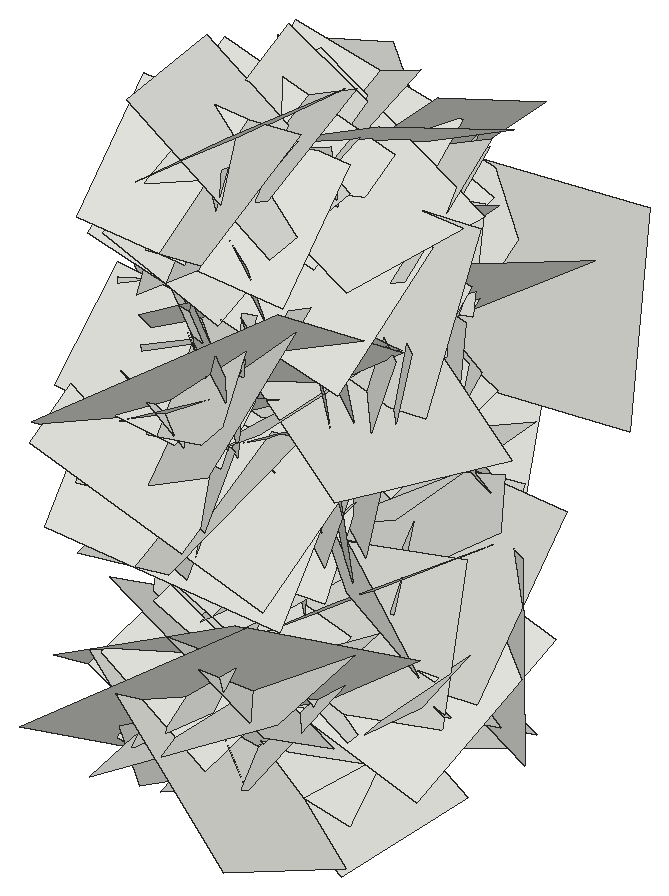
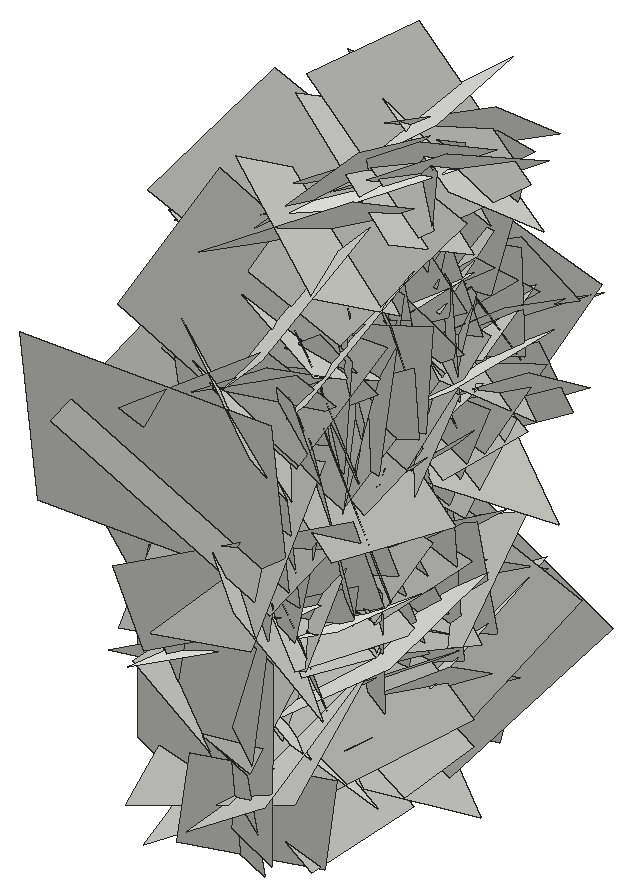
# SketchUp Ruby script. Lengths in inches.
U = 1.inch
M = Sketchup.active_model
def pt(a) = Geom::Point3d.new(a.map { |v| v * U })
def face(e, loops, mat)
  f = e.add_face(loops[0].map { |a| pt(a) })
  loops[1..].each { |l| e.add_face(l.map { |a| pt(a) }).erase! }
  f.material = f.back_material = mat if mat
  f
end
# faces: each face lists its corners as indices into pts; further lists are holes
def faces(e, pts, list, mat = nil) = list.each { |f| face(e, (f[0].is_a?(Array) ? f : [f]).map { |l| l.map { |i| pts[i] } }, mat) }
# xy, xz, yz: faces in a plane at the given z, y or x. An outline is a flat list of corners, or four numbers for a rectangle; further outlines are holes
def ring(l) = l.size == 4 ? [[l[0], l[1]], [l[2], l[1]], [l[2], l[3]], [l[0], l[3]]] : l.each_slice(2).to_a
def flat(e, list, mat, &to3) = list.each { |f| face(e, (f[0].is_a?(Array) ? f : [f]).map { |l| ring(l).map { |u, v| to3.(u, v) } }, mat) }
def xy(e, z, list, mat = nil) = flat(e, list, mat) { |x, y| [x, y, z] }
def xz(e, y, list, mat = nil) = flat(e, list, mat) { |x, z| [x, y, z] }
def yz(e, x, list, mat = nil) = flat(e, list, mat) { |y, z| [x, y, z] }
def lines(e, pts, list) = list.each { |a, b| e.add_line(pt(pts[a]), pt(pts[b])) }
# prism: a flat outline (further loops are holes) pulled along v
def prism(e, loops, v, mat = nil)
  f = face(e, loops, mat); d = Geom::Vector3d.new(v.map { |x| x * U })
  f.pushpull(f.normal.samedirection?(d) ? d.length : -d.length)
end
def box(e, o, s, mat = nil) = prism(e, [[o, [o[0] + s[0], o[1], o[2]], [o[0] + s[0], o[1] + s[1], o[2]], [o[0], o[1] + s[1], o[2]]]], [0, 0, s[2]], mat)
def at(x, y, z, deg = 0) = Geom::Transformation.translation(pt([x, y, z])) * Geom::Transformation.rotation(ORIGIN, Z_AXIS, deg.degrees)
def axes(o, x, y, z) = Geom::Transformation.new([*x, 0, *y, 0, *z, 0, *pt(o).to_a, 1])
def part(name) = M.definitions.add(name)
# library, detail: a bought-in or finely detailed component or shape, given as its bounding box
def library(name, o, s) = part(name).tap { |d| box(d.entities, o, s) }
def detail(e, o, s) = box(e.add_group.entities, o, s)
def put(e, d, t, mat = nil) = e.add_instance(d, t).tap { |i| i.material = mat if mat }
def group(e, t, mat = nil) = e.add_group.tap { |g| g.transformation = t; g.material = mat if mat }.entities
root = M.entities
c1 = part("Component\#6")
p = [[0.01,0,0],[0,3.24,4.54],[4.32,3.24,4.54],[4.33,0,0]]
faces(c1.entities,p,[[0,1,2,3]])
put(root,c1,axes([420.52,211.4,20.36],[-0.11841,0.02386,0.67628],[0.07272,0.6823,-0.01274],[0.7136,-0.06557,0.11352]))
put(root,c1,axes([420.52,208.95,27.68],[-0.1117,0.11156,-0.75397],[-0.06454,-0.75994,-0.10393],[0.80532,-0.04543,-0.11291]))
put(root,c1,axes([420.52,203.96,20.97],[0.02025,-0.24988,0.58047],[-0.03388,0.57961,0.25056],[0.66903,0.03691,-0.00488]))
put(root,c1,axes([420.52,202.42,34.22],[-0.03507,0.56649,-0.26791],[0.06705,-0.26389,-0.56581],[0.66085,0.05684,0.04319]))
put(root,c1,axes([424.49,211.47,22.62],[0.20513,-1.22241,0.07319],[0.04122,0.08019,1.23659],[-1.29742,-0.19072,0.05085]))
put(root,c1,axes([424.49,206.36,33.23],[0.09168,1.1059,0.20164],[0.04784,0.19866,-1.1089],[-1.19063,0.09314,-0.02903]))
put(root,c1,axes([424.49,205.67,24.52],[-0.15369,0.87531,0.08009],[0.01982,0.08422,-0.88666],[-0.9315,-0.14262,-0.03208]))
put(root,c1,axes([424.49,207.21,30.03],[0.00943,-1.01637,-0.0193],[0.00822,-0.01923,1.01638],[-1.07752,-0.00904,0.00758]))
put(root,c1,axes([420.52,204.95,35.05],[0.03568,0.1968,-0.61743],[-0.04358,-0.61637,-0.1987],[0.68554,-0.04943,0.01951]))
put(root,c1,axes([420.52,212.36,26.625],[-0.06935,-0.64087,-0.11796],[0.11905,-0.12787,0.63241],[0.68039,-0.04294,-0.12268]))
put(root,c1,axes([420.52,206.625,39.5],[-0.00312,0.09172,-0.66161],[0.00201,-0.66161,-0.09173],[0.70801,0.00228,-0.00265]))
put(root,c1,axes([420.52,204.22,36.67],[0.08595,0.41822,-0.43473],[-0.01861,-0.43682,-0.42351],[0.63917,-0.06896,0.04613]))
put(root,c1,axes([420.52,202.23,33.91],[0.02493,0.60398,0.49928],[-0.17768,0.49182,-0.58706],[0.81142,0.08914,-0.14389]))
put(root,c1,axes([420.52,200.85,29.625],[-0.04324,0.39016,0.69087],[-0.10275,0.68414,-0.39209],[0.83473,0.10443,-0.01247]))
put(root,c1,axes([420.52,212.78,35.18],[-0.06835,-0.19577,-0.64021],[0.13077,-0.63563,0.18195],[0.69749,0.09999,-0.09685]))
put(root,c1,axes([420.52,211.1,35.2],[0.07899,0.5337,0.27791],[0.02897,0.27674,-0.53878],[0.63716,-0.07875,-0.00996]))
put(root,c1,axes([424.49,202.75,27.49],[0.17368,0.85862,-0.51485],[-0.1903,-0.48804,-0.87105],[-1.04401,0.2318,0.07312]))
put(root,c1,axes([420.52,206.77,29.69],[0.13468,0.0618,0.68245],[-0.14259,0.68282,-0.03679],[0.71222,0.12502,-0.13642]))
put(root,c1,axes([424.49,204.74,34.65],[-0.08046,-0.48471,-0.63269],[-0.12911,-0.62103,0.49039],[-0.83492,0.14274,-0.01486]))
put(root,c1,axes([424.49,210.61,30.96],[-0.02538,-1.03384,0.49264],[0.2847,0.47394,1.00764],[-1.18007,0.13657,0.23251]))
put(root,c1,axes([424.49,212.48,33.12],[-0.02538,-1.03384,0.49264],[0.2847,0.47394,1.00764],[-1.18007,0.13657,0.23251]))
put(root,c1,axes([424.49,201.41,38.375],[0.12316,0.77538,0.57304],[-0.12545,0.58429,-0.76661],[-1.01427,0.02189,0.1644]))
put(root,c1,axes([420.52,207.11,31.75],[-0.23783,0.22127,0.93353],[-0.03566,0.95632,-0.23476],[1.01634,0.08533,0.21022]))
put(root,c1,axes([424.49,210.23,35.31],[-0.06568,0.00099,-0.81141],[-0.08224,-0.81005,0.00494],[-0.85616,0.07773,0.06177]))
put(root,c1,axes([420.52,204.33,34.72],[-0.02793,-0.28222,0.66343],[0.05268,0.66158,0.28341],[0.7624,-0.05605,0.00473]))
put(root,c1,axes([420.52,209.27,26.93],[0.01951,-0.6006,0.29742],[0.06663,0.29777,0.59742],[0.70729,-0.01148,-0.06448]))
put(root,c1,axes([424.49,205.35,34.65],[-0.12302,0.37909,0.72016],[0.00858,0.72795,-0.38188],[-0.86263,-0.04682,-0.1065]))
put(root,c1,axes([424.49,204.65,32.19],[-0.14144,0.68446,-0.34907],[-0.03425,-0.35898,-0.69154],[-0.81371,-0.10387,0.08978]))
put(root,c1,axes([420.52,205,37.54],[0.1597,-0.46751,-0.41946],[-0.05532,-0.43919,0.47075],[0.66349,0.07592,0.14021]))
put(root,c1,axes([420.52,211.91,37.97],[-0.10192,-0.72839,-0.40458],[-0.00784,-0.4065,0.73361],[0.88316,-0.08767,-0.04018]))
put(root,c1,axes([420.52,207.4,37.82],[-0.14382,-0.92009,0.02073],[-0.06912,0.03051,0.92748],[0.97309,-0.13382,0.06894]))
put(root,c1,axes([424.49,206.58,28.49],[-0.01093,-0.51913,0.63451],[-0.10311,0.63085,0.51456],[-0.86287,-0.06881,-0.06953]))
put(root,c1,axes([420.52,201.89,25.36],[0.12511,0.60489,0.30184],[-0.04372,0.31228,-0.60968],[0.71524,-0.08672,-0.09007]))
put(root,c1,axes([420.52,209.37,33.75],[-0.00852,0.3462,-0.76666],[-0.09329,-0.76284,-0.34355],[0.88678,-0.07692,-0.04351]))
put(root,c1,axes([424.49,210.92,34.25],[-0.13403,0.53039,0.57824],[0.04314,0.58935,-0.53168],[-0.83061,-0.05497,-0.12092]))
put(root,c1,axes([420.52,209.14,33.82],[0.16184,0.36707,0.52708],[-0.01835,0.54392,-0.37378],[0.68059,-0.07262,-0.13541]))
put(root,c1,axes([424.49,204.07,39.0625],[0.02986,0.79051,0.40956],[-0.00815,0.40997,-0.79076],[-0.94369,0.02147,0.01979]))
put(root,c1,axes([420.52,207.43,34.16],[0.11276,0.04323,0.70746],[-0.03845,0.71477,-0.03823],[0.75032,0.03013,-0.10828]))
put(root,c1,axes([424.49,200.125,30.08],[0.25415,0.9144,0.59243],[0.00684,0.60541,-0.93704],[-1.1549,0.20481,0.12483]))
put(root,c1,axes([424.49,209.72,22.08],[0.18138,-0.91546,-0.54155],[0.07402,-0.53767,0.93095],[-1.12504,-0.18297,-0.02606]))
put(root,c1,axes([424.49,208.86,27.22],[0.22907,0.58895,0.94038],[0.09031,0.94642,-0.61231],[-1.17269,0.18793,0.13653]))
put(root,c1,axes([424.49,209.27,26.87],[-0.02942,-0.98917,0.00062],[0.2303,-0.00549,0.9654],[-1.02292,0.02721,0.21733]))
put(root,c1,axes([420.52,202.89,32.22],[-0.0211,0.0618,0.84202],[-0.01452,0.84212,-0.06213],[0.89482,0.01512,0.01885]))
put(root,c1,axes([424.49,210.17,27.25],[-0.0389,-0.19659,0.74237],[-0.03773,0.74285,0.19496],[-0.81316,-0.02506,-0.04456]))
put(root,c1,axes([424.49,209.1,25.86],[0.06992,-0.92649,-0.30548],[0.11921,-0.29692,0.92479],[-1.02719,-0.09753,0.08653]))
put(root,c1,axes([420.52,209.1,25.86],[-0.06992,-0.92649,-0.30548],[-0.11921,-0.29692,0.92479],[1.02719,-0.09753,0.08653]))
put(root,c1,axes([420.52,210.17,27.25],[0.0389,-0.19659,0.74237],[0.03773,0.74285,0.19496],[0.81316,-0.02506,-0.04456]))
put(root,c1,axes([424.49,202.89,32.22],[0.0211,0.0618,0.84202],[0.01452,0.84212,-0.06213],[-0.89482,0.01512,0.01885]))
put(root,c1,axes([420.52,209.27,26.87],[0.02942,-0.98917,0.00062],[-0.2303,-0.00549,0.9654],[1.02292,0.02721,0.21733]))
put(root,c1,axes([420.52,208.86,27.22],[-0.22907,0.58895,0.94038],[-0.09031,0.94642,-0.61231],[1.17269,0.18793,0.13653]))
put(root,c1,axes([420.52,209.72,22.08],[-0.18138,-0.91546,-0.54155],[-0.07402,-0.53767,0.93095],[1.12504,-0.18297,-0.02606]))
put(root,c1,axes([420.52,200.125,30.08],[-0.25415,0.9144,0.59243],[-0.00684,0.60541,-0.93704],[1.1549,0.20481,0.12483]))
put(root,c1,axes([424.49,207.43,34.16],[-0.11276,0.04323,0.70746],[0.03845,0.71477,-0.03823],[-0.75032,0.03013,-0.10828]))
put(root,c1,axes([420.52,204.07,39.0625],[-0.02986,0.79051,0.40956],[0.00815,0.40997,-0.79076],[0.94369,0.02147,0.01979]))
put(root,c1,axes([424.49,209.14,33.82],[-0.16184,0.36707,0.52708],[0.01835,0.54392,-0.37378],[-0.68059,-0.07262,-0.13541]))
put(root,c1,axes([420.52,210.92,34.25],[0.13403,0.53039,0.57824],[-0.04314,0.58935,-0.53168],[0.83061,-0.05497,-0.12092]))
put(root,c1,axes([424.49,209.37,33.75],[0.00852,0.3462,-0.76666],[0.09329,-0.76284,-0.34355],[-0.88678,-0.07692,-0.04351]))
put(root,c1,axes([424.49,201.89,25.36],[-0.12511,0.60489,0.30184],[0.04372,0.31228,-0.60968],[-0.71524,-0.08672,-0.09007]))
put(root,c1,axes([420.52,206.58,28.49],[0.01093,-0.51913,0.63451],[0.10311,0.63085,0.51456],[0.86287,-0.06881,-0.06953]))
put(root,c1,axes([424.49,207.4,37.82],[0.14382,-0.92009,0.02073],[0.06912,0.03051,0.92748],[-0.97309,-0.13382,0.06894]))
put(root,c1,axes([424.49,211.91,37.97],[0.10192,-0.72839,-0.40458],[0.00784,-0.4065,0.73361],[-0.88316,-0.08767,-0.04018]))
put(root,c1,axes([424.49,205,37.54],[-0.1597,-0.46751,-0.41946],[0.05532,-0.43919,0.47075],[-0.66349,0.07592,0.14021]))
put(root,c1,axes([420.52,204.65,32.19],[0.14144,0.68446,-0.34907],[0.03425,-0.35898,-0.69154],[0.81371,-0.10387,0.08978]))
put(root,c1,axes([420.52,205.35,34.65],[0.12302,0.37909,0.72016],[-0.00858,0.72795,-0.38188],[0.86263,-0.04682,-0.1065]))
put(root,c1,axes([424.49,209.27,26.93],[-0.01951,-0.6006,0.29742],[-0.06663,0.29777,0.59742],[-0.70729,-0.01148,-0.06448]))
put(root,c1,axes([424.49,204.33,34.72],[0.02793,-0.28222,0.66343],[-0.05268,0.66158,0.28341],[-0.7624,-0.05605,0.00473]))
put(root,c1,axes([420.52,210.23,35.31],[0.06568,0.00099,-0.81141],[0.08224,-0.81005,0.00494],[0.85616,0.07773,0.06177]))
put(root,c1,axes([424.49,207.11,31.75],[0.23783,0.22127,0.93353],[0.03566,0.95632,-0.23476],[-1.01634,0.08533,0.21022]))
put(root,c1,axes([420.52,201.41,38.375],[-0.12316,0.77538,0.57304],[0.12545,0.58429,-0.76661],[1.01427,0.02189,0.1644]))
put(root,c1,axes([420.52,210.61,30.96],[0.02538,-1.03384,0.49264],[-0.2847,0.47394,1.00764],[1.18007,0.13657,0.23251]))
put(root,c1,axes([420.52,212.48,33.12],[0.02538,-1.03384,0.49264],[-0.2847,0.47394,1.00764],[1.18007,0.13657,0.23251]))
put(root,c1,axes([420.52,204.74,34.65],[0.08046,-0.48471,-0.63269],[0.12911,-0.62103,0.49039],[0.83492,0.14274,-0.01486]))
put(root,c1,axes([424.49,206.77,29.69],[-0.13468,0.0618,0.68245],[0.14259,0.68282,-0.03679],[-0.71222,0.12502,-0.13642]))
put(root,c1,axes([420.52,202.75,27.49],[-0.17368,0.85862,-0.51485],[0.1903,-0.48804,-0.87105],[1.04401,0.2318,0.07312]))
put(root,c1,axes([424.49,211.1,35.2],[-0.07899,0.5337,0.27791],[-0.02897,0.27674,-0.53878],[-0.63716,-0.07875,-0.00996]))
put(root,c1,axes([424.49,212.78,35.18],[0.06835,-0.19577,-0.64021],[-0.13077,-0.63563,0.18195],[-0.69749,0.09999,-0.09685]))
put(root,c1,axes([424.49,200.85,29.625],[0.04324,0.39016,0.69087],[0.10275,0.68414,-0.39209],[-0.83473,0.10443,-0.01247]))
put(root,c1,axes([424.49,202.23,33.91],[-0.02493,0.60398,0.49928],[0.17768,0.49182,-0.58706],[-0.81142,0.08914,-0.14389]))
put(root,c1,axes([424.49,204.22,36.67],[-0.08595,0.41822,-0.43473],[0.01861,-0.43682,-0.42351],[-0.63917,-0.06896,0.04613]))
put(root,c1,axes([424.49,206.625,39.5],[0.00312,0.09172,-0.66161],[-0.00201,-0.66161,-0.09173],[-0.70801,0.00228,-0.00265]))
put(root,c1,axes([424.49,212.36,26.625],[0.06935,-0.64087,-0.11796],[-0.11905,-0.12787,0.63241],[-0.68039,-0.04294,-0.12268]))
put(root,c1,axes([424.49,204.95,35.05],[-0.03568,0.1968,-0.61743],[0.04358,-0.61637,-0.1987],[-0.68554,-0.04943,0.01951]))
put(root,c1,axes([420.52,207.21,30.03],[-0.00943,-1.01637,-0.0193],[-0.00822,-0.01923,1.01638],[1.07752,-0.00904,0.00758]))
put(root,c1,axes([420.52,205.67,24.52],[0.15369,0.87531,0.08009],[-0.01982,0.08422,-0.88666],[0.9315,-0.14262,-0.03208]))
put(root,c1,axes([420.52,206.36,33.23],[-0.09168,1.1059,0.20164],[-0.04784,0.19866,-1.1089],[1.19063,0.09314,-0.02903]))
put(root,c1,axes([420.52,211.47,22.62],[-0.20513,-1.22241,0.07319],[-0.04122,0.08019,1.23659],[1.29742,-0.19072,0.05085]))
put(root,c1,axes([424.49,202.42,34.22],[0.03507,0.56649,-0.26791],[-0.06705,-0.26389,-0.56581],[-0.66085,0.05684,0.04319]))
put(root,c1,axes([424.49,203.96,20.97],[-0.02025,-0.24988,0.58047],[0.03388,0.57961,0.25056],[-0.66903,0.03691,-0.00488]))
put(root,c1,axes([424.49,208.95,27.68],[0.1117,0.11156,-0.75397],[0.06454,-0.75994,-0.10393],[-0.80532,-0.04543,-0.11291]))
put(root,c1,axes([424.49,211.4,20.36],[0.11841,0.02386,0.67628],[-0.07272,0.6823,-0.01274],[-0.7136,-0.06557,0.11352]))
put(root,c1,axes([420.52,209.77,25.57],[-0.04769,1.02209,-0.46416],[-0.05126,-0.46587,-1.02116],[1.18879,0.02092,-0.06265]))
put(root,c1,axes([420.52,212.41,27.7],[0.11035,-0.46639,-0.85158],[-0.0233,-0.85737,0.46687],[1.02892,0.03061,0.1019]))
put(root,c1,axes([424.49,210.37,37.54],[0.0852,-0.7988,-0.26142],[0.21653,-0.23617,0.78446],[-0.8642,-0.13792,0.17078]))
put(root,c1,axes([424.49,207.84,29.22],[0.13906,-0.51177,-0.49755],[-0.00544,-0.50655,0.51967],[-0.75658,-0.09042,-0.09518]))
put(root,c1,axes([420.52,211.63,27.44],[0.13698,0.50835,-0.7639],[0.02564,-0.77306,-0.51036],[0.97231,-0.05123,0.12108]))
put(root,c1,axes([420.52,212.85,24.81],[-0.10314,-0.72888,-0.73382],[0.20394,-0.73695,0.70648],[1.07722,0.06973,-0.20401]))
put(root,c1,axes([420.52,211.43,33.78],[-0.23599,-0.36182,-1.29322],[-0.09706,-1.30373,0.38052],[1.42014,-0.14923,-0.18889]))
put(root,c1,axes([420.52,199.54,32.72],[-0.14681,1.15124,0.44909],[-0.05729,0.44582,-1.15954],[1.30862,0.14867,-0.00039]))
put(root,c1,axes([420.52,206.07,20.81],[-0.31441,-1.20333,0.63493],[-0.01893,0.65323,1.22967],[1.44208,-0.25378,0.15457]))
put(root,c1,axes([420.52,208.01,36.375],[-0.10923,0.38133,-1.06486],[0.05778,-1.06635,-0.38714],[1.19755,0.08623,-0.07845]))
put(root,c1,axes([420.52,212.99,32.26],[0.05541,-0.21084,-0.92918],[0.15034,-0.91849,0.21639],[0.99872,0.14996,0.01898]))
put(root,c1,axes([420.52,205.46,33.43],[0.14097,0.63084,0.7943],[-0.06243,0.80455,-0.62912],[1.07339,-0.03606,-0.14091]))
put(root,c1,axes([420.52,207.91,30.98],[-0.03881,-0.77727,0.6188],[0.26695,0.59174,0.75817],[1.01873,-0.18467,-0.1751]))
put(root,c1,axes([424.49,206,31.6],[0.1462,-0.08624,0.716],[0.07336,0.72719,0.07426],[-0.76092,0.05354,0.14472]))
put(root,c1,axes([424.49,210.56,30.82],[0.08988,0.23539,0.56706],[-0.00516,0.57268,-0.23699],[-0.65079,0.02797,0.0802]))
put(root,c1,axes([420.52,206.55,33.15],[0.00164,-0.95203,-0.71322],[-0.09471,-0.7113,0.94927],[1.25737,-0.05234,0.07244]))
put(root,c1,axes([420.52,206.8125,26.89],[-0.15204,1.11982,0.24611],[0.19339,0.26716,-1.10927],[1.19986,0.09884,0.20998]))
put(root,c1,axes([420.52,211.99,33.59],[-0.13241,-0.25962,-1.28668],[-0.09489,-1.2878,0.26854],[1.38813,-0.1128,-0.10438]))
put(root,c1,axes([420.52,206.95,24.98],[0.09414,0.39654,1.07266],[-0.12922,1.07305,-0.38659],[1.20532,0.08407,-0.12522]))
put(root,c1,axes([424.49,202.49,32.61],[0.11645,-0.17214,0.59947],[0.01233,0.60916,0.17278],[-0.661,-0.01896,0.10883]))
put(root,c1,axes([420.52,205.38,23.16],[0.04798,1.09948,0.05597],[0.01409,0.05547,-1.10036],[1.16688,-0.04588,0.01099]))
put(root,c1,axes([420.52,210.75,36.02],[-0.14272,-1.0645,0.43866],[0.22696,0.41079,1.0626],[1.19913,-0.20445,-0.14891]))
put(root,c1,axes([420.52,208.81,31.45],[-0.04602,0.84125,-1.04893],[-0.18208,-1.04435,-0.83047],[1.4136,-0.10713,-0.14111]))
put(root,c1,axes([420.52,213.59,29.33],[0.10669,0.07311,-1.12569],[-0.06812,-1.12796,-0.079],[1.19381,-0.0709,0.09609]))
put(root,c1,axes([420.52,201.95,25.76],[0.02109,1.10253,-0.4508],[-0.04504,-0.44992,-1.10225],[1.2618,-0.03449,-0.03181]))
put(root,c1,axes([420.52,213.06,27.02],[-0.109,-1.16412,-0.17966],[0.1638,-0.19212,1.15639],[1.23778,-0.07709,-0.16885]))
put(root,c1,axes([420.52,201.85,37.73],[-0.10519,1.13817,0.58904],[-0.00109,0.59073,-1.14161],[1.35845,0.08861,0.0447]))
put(root,c1,axes([420.52,204.59,30.02],[-0.04301,-1.09683,0.72238],[-0.12053,0.72294,1.0913],[1.38692,0.02882,0.11724]))
put(root,c1,axes([420.52,209.74,33.23],[0.15201,0.07034,-1.21602],[-0.20156,-1.20811,-0.09231],[1.2753,-0.19933,0.13035]))
put(root,c1,axes([420.52,208.94,26.04],[-0.1299,1.02121,-0.60997],[0.25035,-0.5801,-1.01865],[1.23578,0.22487,0.14225]))
put(root,c1,axes([420.52,213.71,29.11],[-0.07729,-1.24842,0.49404],[-0.03127,0.49613,1.24937],[1.42283,-0.05691,0.0543]))
put(root,c1,axes([420.52,211.375,32.78],[-0.08242,0.8278,-0.94283],[0.12426,-0.93571,-0.83122],[1.32412,0.13934,0.01932]))
put(root,c1,axes([420.52,211.85,35.53],[0.11979,-0.95717,-0.48165],[0.13908,-0.46832,0.96146],[1.12727,0.15949,-0.06744]))
put(root,c1,axes([420.52,203.71,22.72],[-0.0324,0.32539,1.27516],[0.00551,1.27553,-0.32536],[1.39498,0.00251,0.0309]))
put(root,c1,axes([420.52,205.99,22.98],[0.14358,-1.11124,-0.06865],[0.09474,-0.05808,1.11649],[1.17635,0.14031,-0.08154]))
put(root,c1,axes([420.52,205.63,39.17],[0.17317,1.06099,0.10432],[0.22006,0.07185,-1.05594],[1.10844,-0.18002,0.19334]))
put(root,c1,axes([420.52,205.46,24.09],[0.08024,0.04196,1.34674],[-0.06239,1.34768,-0.03868],[1.42687,0.05657,-0.07742]))
put(root,c1,axes([420.52,204.65,33.57],[0.11682,0.36237,1.1463],[0.15256,1.13885,-0.37385],[1.26518,-0.17079,-0.06076]))
put(root,c1,axes([420.52,211.92,20.51],[0.20622,-1.25394,-0.15944],[-0.06822,-0.17093,1.26581],[1.33814,0.18453,0.0891]))
put(root,c1,axes([420.52,213.57,27.56],[-0.01798,0.03957,-1.39555],[0.22262,-1.3797,-0.04168],[1.46303,0.21042,-0.01081]))
put(root,c1,axes([420.52,205.51,24.88],[0.13882,1.11155,0.63897],[0.19603,0.6192,-1.11507],[1.34484,-0.205,0.09658]))
put(root,c1,axes([420.17,214.11,35.21],[0.07772,-0.27644,-1.33377],[0.91911,-1.02064,0.2592],[1.11351,0.86175,-0.12086]))
put(root,c1,axes([420.52,205.05,35.75],[0.23328,1.34713,-0.22992],[0.05022,-0.24027,-1.36238],[1.44774,-0.20874,0.08431]))
put(root,c1,axes([420.52,206.12,25.83],[0.28838,0.48251,1.20317],[0.13396,1.21365,-0.51529],[1.36755,-0.22063,-0.20324]))
